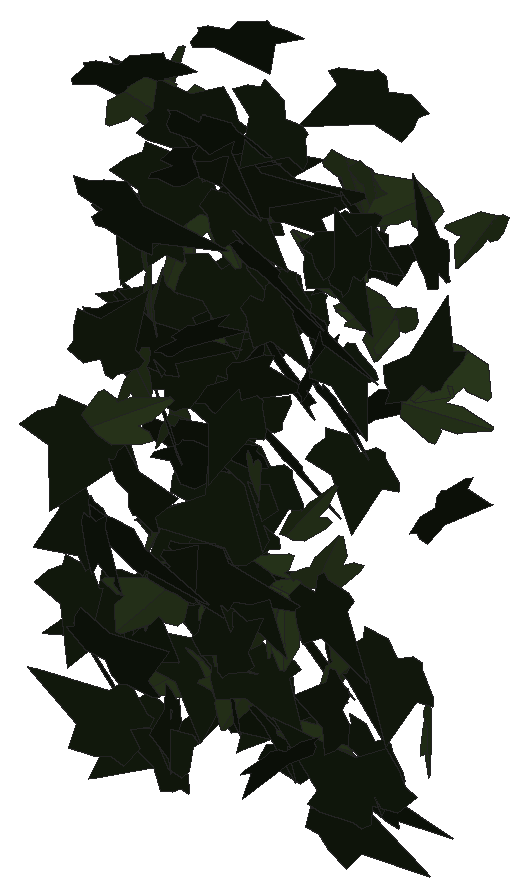
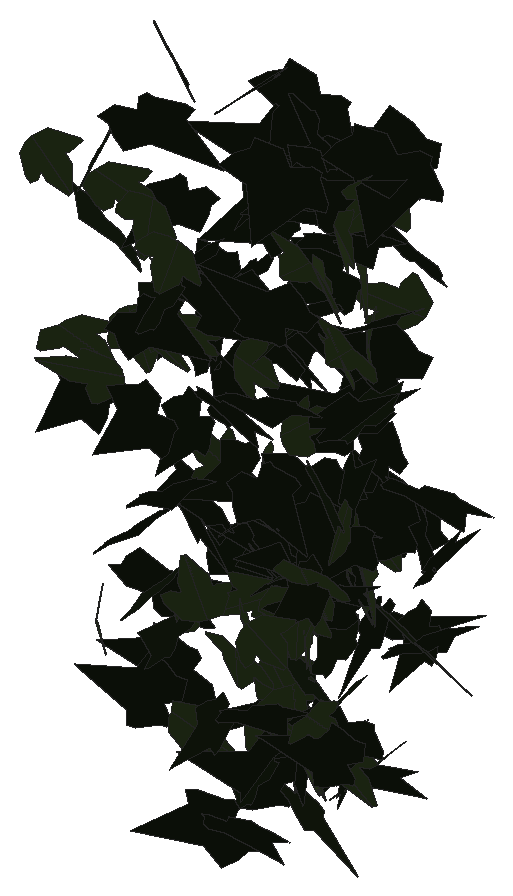
# SketchUp Ruby script. Lengths in inches.
U = 1.inch
M = Sketchup.active_model
def pt(a) = Geom::Point3d.new(a.map { |v| v * U })
def face(e, loops, mat)
  f = e.add_face(loops[0].map { |a| pt(a) })
  loops[1..].each { |l| e.add_face(l.map { |a| pt(a) }).erase! }
  f.material = f.back_material = mat if mat
  f
end
# faces: each face lists its corners as indices into pts; further lists are holes
def faces(e, pts, list, mat = nil) = list.each { |f| face(e, (f[0].is_a?(Array) ? f : [f]).map { |l| l.map { |i| pts[i] } }, mat) }
# xy, xz, yz: faces in a plane at the given z, y or x. An outline is a flat list of corners, or four numbers for a rectangle; further outlines are holes
def ring(l) = l.size == 4 ? [[l[0], l[1]], [l[2], l[1]], [l[2], l[3]], [l[0], l[3]]] : l.each_slice(2).to_a
def flat(e, list, mat, &to3) = list.each { |f| face(e, (f[0].is_a?(Array) ? f : [f]).map { |l| ring(l).map { |u, v| to3.(u, v) } }, mat) }
def xy(e, z, list, mat = nil) = flat(e, list, mat) { |x, y| [x, y, z] }
def xz(e, y, list, mat = nil) = flat(e, list, mat) { |x, z| [x, y, z] }
def yz(e, x, list, mat = nil) = flat(e, list, mat) { |y, z| [x, y, z] }
def lines(e, pts, list) = list.each { |a, b| e.add_line(pt(pts[a]), pt(pts[b])) }
# prism: a flat outline (further loops are holes) pulled along v
def prism(e, loops, v, mat = nil)
  f = face(e, loops, mat); d = Geom::Vector3d.new(v.map { |x| x * U })
  f.pushpull(f.normal.samedirection?(d) ? d.length : -d.length)
end
def box(e, o, s, mat = nil) = prism(e, [[o, [o[0] + s[0], o[1], o[2]], [o[0] + s[0], o[1] + s[1], o[2]], [o[0], o[1] + s[1], o[2]]]], [0, 0, s[2]], mat)
def at(x, y, z, deg = 0) = Geom::Transformation.translation(pt([x, y, z])) * Geom::Transformation.rotation(ORIGIN, Z_AXIS, deg.degrees)
def axes(o, x, y, z) = Geom::Transformation.new([*x, 0, *y, 0, *z, 0, *pt(o).to_a, 1])
def part(name) = M.definitions.add(name)
# library, detail: a bought-in or finely detailed component or shape, given as its bounding box
def library(name, o, s) = part(name).tap { |d| box(d.entities, o, s) }
def detail(e, o, s) = box(e.add_group.entities, o, s)
def put(e, d, t, mat = nil) = e.add_instance(d, t).tap { |i| i.material = mat if mat }
def group(e, t, mat = nil) = e.add_group.tap { |g| g.transformation = t; g.material = mat if mat }.entities
root = M.entities
M.materials.add("1026 AP 7946 SUNNY SIDE UP").color = [254, 231, 186]
M.materials.add("efeu1").color = [18, 25, 13]
M.materials.add("efeu2").color = [43, 57, 29]
c1 = part("ivyleaf_9")
p = [[1.54,2.16,1.25],[1.36,2.04,1.19],[-0.21,0.99,0.68],[-0.71,1.11,0.82],[-0.85,0.86,0.67],[-0.8,0.17,0.21],
  [-0.9,-0.01,0.1],[-0.67,-0.16,-0.02],[-0.08,-0.08,-0.05],[-0.03,-0.6,-0.4],[0.65,-0.88,-0.66],[0.83,-0.6,-0.49],
  [1.29,-0.42,-0.43],[1.8125,-0.07,-0.26],[1.21,0.44,0.15]]
faces(c1.entities,p,[[0,1,2,3,4,5,6,7,8,9,10,11,12,13,14]],"efeu1")
c2 = part("ivyleaf_10")
p = [[0,0.5,-0.03],[-0.0625,2.02,-0.43],[-0.19,2.01,-0.46],[-0.54,1.05,-0.29],[-0.52,0.625,-0.18],[-0.83,0.76,-0.28],
  [-1.16,0.64,-0.33],[-1.15,0.33,-0.24],[-0.77,-0.39,0.02],[-0.3,-0.51,0.16],[0.04,-0.48,0.23],[-0.02,2.01,-0.4375],
  [-0.06,2.01,-0.43],[0.04,-0.49,0.23],[0.67,-0.49,0.14],[1.38,0.36,-0.2],[1.375,0.51,-0.24],[0.81,0.65,-0.19],
  [0.62,0.59,-0.15],[0.6,1.09,-0.28],[0.5,1.23,-0.31]]
faces(c2.entities,p,[[0,1,2,3,4,5,6,7,8,9,10],[11,12,0,13,14,15,16,17,18,19,20]],"efeu2")
put(root,c1,axes([146.34,207.53,282.68],[-0.11458,-0.05735,0.44093],[0.46004,-0.32624,0.00437],[0.50012,0.28696,0.097]),"1026 AP 7946 SUNNY SIDE UP")
put(root,c2,axes([146.33,207.56,286.51],[-0.17998,-0.16825,0.34031],[0.22211,0.30092,0.20948],[-0.54038,0.17972,-0.02724]),"1026 AP 7946 SUNNY SIDE UP")
put(root,c1,axes([146.125,207.66,287.49],[-0.35598,0.26157,0.18173],[0.20681,-0.1171,0.35508],[0.44949,0.26103,-0.01945]),"1026 AP 7946 SUNNY SIDE UP")
put(root,c1,axes([146.3,207.96,281.36],[-0.37631,-0.28963,-0.13625],[-0.16376,-0.08298,0.38565],[-0.47198,0.25971,-0.02517]),"1026 AP 7946 SUNNY SIDE UP")
put(root,c1,axes([149.12,208.05,281.89],[-0.08149,0.34391,-0.18116],[0.03588,-0.17637,-0.35931],[-0.6077,-0.05653,0.00308]),"1026 AP 7946 SUNNY SIDE UP")
put(root,c1,axes([145.72,208.29,289.42],[0.35847,-0.07858,0.41361],[0.57645,-0.16589,-0.2486],[0.28705,0.43128,-0.01728]),"1026 AP 7946 SUNNY SIDE UP")
put(root,c2,axes([146.45,208.48,283.31],[-0.42331,-0.17634,0.21143],[-0.22299,-0.15626,-0.32925],[0.36376,-0.30099,0.04422]),"1026 AP 7946 SUNNY SIDE UP")
put(root,c1,axes([145.78,208.74,284.66],[0.02851,0.01116,0.39344],[0.25825,-0.34537,0.00034],[0.54233,0.16388,-0.02085]),"1026 AP 7946 SUNNY SIDE UP")
put(root,c1,axes([145.14,208.58,282.01],[0.47396,-0.14013,-0.18759],[-0.2741,0.05421,-0.34142],[0.23386,0.34755,-0.01997]),"1026 AP 7946 SUNNY SIDE UP")
put(root,c1,axes([144.9375,208.9,283.82],[0.04348,-0.10932,-0.40963],[0.628,-0.08975,0.0536],[-0.15764,-0.38772,0.10052]),"1026 AP 7946 SUNNY SIDE UP")
put(root,c1,axes([149.72,208.57,282.58],[-0.10359,-0.01043,-0.40068],[-0.60269,0.06915,0.06539],[0.10455,0.38831,-0.02006]),"1026 AP 7946 SUNNY SIDE UP")
put(root,c1,axes([145.39,208.82,283.78],[0.45446,-0.18086,0.27953],[0.33247,-0.17388,-0.35111],[0.39211,0.35705,-0.02627]),"1026 AP 7946 SUNNY SIDE UP")
put(root,c1,axes([150.02,208.46,289.85],[-0.01429,0.13954,0.37864],[-0.11431,0.3599,-0.14082],[-0.60633,-0.07114,0.01762]),"1026 AP 7946 SUNNY SIDE UP")
put(root,c1,axes([144.58,209.23,283.5],[-0.14243,-0.16436,0.36457],[-0.23731,-0.32131,-0.1949],[0.56724,-0.17569,0.01001]),"1026 AP 7946 SUNNY SIDE UP")
put(root,c1,axes([149.98,208.89,281.04],[0.00757,0.06868,0.46089],[-0.63803,0.19805,-0.02569],[-0.314,-0.40076,0.06331]),"1026 AP 7946 SUNNY SIDE UP")
put(root,c1,axes([146.72,208.68,287.51],[0.29215,0.21801,0.26175],[0.23418,0.20485,-0.29351],[-0.46982,0.23767,0.01647]),"1026 AP 7946 SUNNY SIDE UP")
put(root,c2,axes([145.72,208.93,286.54],[0.00431,-0.31487,-0.22093],[0.08161,0.21099,-0.3199],[0.59185,-0.0268,0.04572]),"1026 AP 7946 SUNNY SIDE UP")
put(root,c2,axes([146.13,208.85,287.75],[-0.04394,0.12117,0.3695],[-0.38677,0.2667,-0.11121],[-0.45118,-0.24042,0.05935]),"1026 AP 7946 SUNNY SIDE UP")
put(root,c1,axes([144.625,209.42,282.35],[-0.27092,-0.36562,0.1011],[-0.02765,-0.10225,-0.41607],[0.59547,-0.17109,0.02668]),"1026 AP 7946 SUNNY SIDE UP")
put(root,c1,axes([147.29,209.32,286.38],[-0.51987,-0.00879,-0.25074],[0.37992,-0.06273,-0.33623],[-0.04748,-0.4057,0.05499]),"1026 AP 7946 SUNNY SIDE UP")
put(root,c1,axes([145.4,209.21,282.45],[-0.57652,0.24626,0.03011],[-0.06689,-0.01359,-0.45366],[-0.3839,-0.36745,0.03384]),"1026 AP 7946 SUNNY SIDE UP")
put(root,c1,axes([144.55,209.45,284.92],[-0.58467,-0.19631,-0.09866],[0.17905,-0.01539,-0.42803],[0.29219,-0.38338,0.06487]),"1026 AP 7946 SUNNY SIDE UP")
put(root,c1,axes([149,209.34,280.32],[0.20714,-0.07694,-0.41271],[0.594,0.18077,0.09336],[0.24029,-0.38055,0.12497]),"1026 AP 7946 SUNNY SIDE UP")
put(root,c1,axes([145.63,209.11,282.32],[0.18332,-0.11785,-0.43679],[-0.43229,0.32209,-0.16849],[0.539,0.29841,0.01342]),"1026 AP 7946 SUNNY SIDE UP")
put(root,c2,axes([145.73,209.52,282.94],[0.31557,-0.29001,0.16499],[0.11435,-0.14609,-0.36353],[0.50952,0.21241,-0.0206]),"1026 AP 7946 SUNNY SIDE UP")
put(root,c1,axes([146.67,209.25,290.72],[0.63521,0.10103,-0.0912],[-0.12008,-0.06027,-0.42745],[-0.17449,0.40927,-0.03784]),"1026 AP 7946 SUNNY SIDE UP")
put(root,c1,axes([149.5,209.64,281.48],[0.02809,-0.33997,0.1459],[0.00465,-0.14359,-0.35153],[0.58025,0.01761,-0.00424]),"1026 AP 7946 SUNNY SIDE UP")
put(root,c1,axes([145.15,209.4,286.65],[0.18157,-0.04685,0.45099],[0.65903,-0.12779,-0.12865],[0.21335,0.43461,0.01358]),"1026 AP 7946 SUNNY SIDE UP")
put(root,c1,axes([146.45,209.58,290.3125],[-0.01147,-0.02937,-0.4212],[0.64309,0.02428,-0.00918],[0.03909,-0.40803,0.02737]),"1026 AP 7946 SUNNY SIDE UP")
put(root,c1,axes([148.47,209.62,283.52],[-0.07092,-0.10751,-0.41748],[0.65506,0.02896,-0.0556],[0.06549,-0.40611,0.10401]),"1026 AP 7946 SUNNY SIDE UP")
put(root,c1,axes([147.11,209.5625,288.78],[0.62479,-0.1759,0.05333],[0.05181,-0.05544,-0.44635],[0.28407,0.39698,-0.03588]),"1026 AP 7946 SUNNY SIDE UP")
put(root,c1,axes([146.76,209.52,282.07],[-0.22697,0.28518,0.24524],[0.20555,-0.19821,0.32736],[0.54502,0.19352,-0.02133]),"1026 AP 7946 SUNNY SIDE UP")
put(root,c1,axes([146.93,209.49,289.71],[0.24049,0.01486,0.39247],[0.59898,-0.02046,-0.15688],[0.02118,0.40993,-0.01965]),"1026 AP 7946 SUNNY SIDE UP")
put(root,c1,axes([146.96,209.52,289.54],[0.21222,-0.27332,-0.30954],[-0.16993,0.27935,-0.31178],[0.61379,0.17184,0.02071]),"1026 AP 7946 SUNNY SIDE UP")
put(root,c1,axes([146.2,209.55,283.26],[0.31222,0.08967,-0.4258],[0.53074,0.24246,0.22238],[0.40201,-0.38974,0.0371]),"1026 AP 7946 SUNNY SIDE UP")
put(root,c1,axes([147.13,209.32,286.7],[-0.04177,0.09236,-0.41009],[-0.08616,0.39503,0.10037],[0.63756,0.05943,-0.0133]),"1026 AP 7946 SUNNY SIDE UP")
put(root,c1,axes([146.06,209.4,283.25],[0.13493,0.18267,-0.38061],[0.16325,0.35672,0.20804],[0.62868,-0.13184,0.02766]),"1026 AP 7946 SUNNY SIDE UP")
put(root,c1,axes([149.62,209.97,282.71],[-0.11211,-0.40787,0.12598],[-0.02984,-0.12317,-0.42727],[0.66993,-0.07374,0.00205]),"1026 AP 7946 SUNNY SIDE UP")
put(root,c1,axes([147.5,210.05,290.75],[-0.22523,-0.2758,0.27981],[-0.10509,-0.26931,-0.31779],[0.60128,-0.15038,0.04927]),"1026 AP 7946 SUNNY SIDE UP")
put(root,c1,axes([145.6,209.93,279.74],[0.06804,-0.34981,-0.06883],[0.02076,-0.06368,0.36271],[-0.55903,-0.04494,0.00509]),"1026 AP 7946 SUNNY SIDE UP")
put(root,c1,axes([145.41,209.98,280.12],[-0.50858,-0.1978,0.12312],[-0.13387,-0.0912,-0.38973],[0.33882,-0.33294,0.03083]),"1026 AP 7946 SUNNY SIDE UP")
put(root,c1,axes([146.71,209.86,283.25],[-0.1452,-0.07776,-0.41071],[0.61179,0.09888,-0.11226],[0.18098,-0.39665,0.04998]),"1026 AP 7946 SUNNY SIDE UP")
put(root,c2,axes([145.42,209.74,283.48],[0.18911,-0.35834,-0.13358],[-0.06344,0.12109,-0.38869],[0.59476,0.12686,0.00101]),"1026 AP 7946 SUNNY SIDE UP")
put(root,c2,axes([145.02,210.0625,287.42],[0.06252,-0.10645,0.39735],[0.40863,-0.28864,-0.11118],[0.4796,0.25981,0.04294]),"1026 AP 7946 SUNNY SIDE UP")
put(root,c1,axes([147.42,209.76,287.85],[0.18573,-0.26181,-0.23419],[-0.13911,0.20783,-0.29465],[0.52557,0.14753,0.00477]),"1026 AP 7946 SUNNY SIDE UP")
put(root,c1,axes([145.58,210.13,289.125],[-0.43309,-0.29961,-0.01191],[0.03845,-0.00912,-0.41857],[0.46979,-0.27545,0.02328]),"1026 AP 7946 SUNNY SIDE UP")
put(root,c1,axes([146.95,210.1,284],[-0.51564,-0.01116,0.29046],[-0.43109,-0.09008,-0.33262],[0.1054,-0.42303,0.06057]),"1026 AP 7946 SUNNY SIDE UP")
put(root,c1,axes([145.42,210.21,279.96],[-0.0198,-0.03089,0.41541],[-0.17984,-0.38688,-0.03646],[0.61024,-0.11501,0.00274]),"1026 AP 7946 SUNNY SIDE UP")
put(root,c2,axes([147.93,209.87,284.35],[-0.00619,-0.29915,0.21667],[0.02685,0.21166,0.30921],[-0.57592,0.01309,0.01209]),"1026 AP 7946 SUNNY SIDE UP")
put(root,c2,axes([148.33,210.28,281.96],[-0.01656,0.04386,0.39384],[0.2344,-0.35184,0.04379],[0.5574,0.14926,-0.00671]),"1026 AP 7946 SUNNY SIDE UP")
put(root,c1,axes([145.85,209.71,289.59],[0.40829,0.1815,0.33611],[0.39514,0.20724,-0.32462],[-0.43223,0.3609,0.02072]),"1026 AP 7946 SUNNY SIDE UP")
put(root,c1,axes([145.73,210.3125,283.14],[-0.39581,-0.23494,0.13572],[-0.10522,-0.12198,-0.35297],[0.41132,-0.25728,0.04031]),"1026 AP 7946 SUNNY SIDE UP")
put(root,c1,axes([150.28,209.74,287.62],[-0.51887,0.3022,-0.16496],[-0.1532,0.1327,0.46069],[0.5168,0.34275,-0.02905]),"1026 AP 7946 SUNNY SIDE UP")
put(root,c1,axes([144.82,210.43,286.4],[-0.04605,-0.30692,0.30359],[0.12614,-0.2958,-0.30907],[0.65899,0.03517,0.08037]),"1026 AP 7946 SUNNY SIDE UP")
put(root,c1,axes([144.8,210.4,288.04],[-0.26732,-0.32537,0.1346],[-0.00014,-0.14716,-0.37326],[0.55241,-0.15749,0.06504]),"1026 AP 7946 SUNNY SIDE UP")
put(root,c1,axes([147.67,210.15,287.62],[0.49542,-0.16371,0.15009],[0.17755,-0.09928,-0.36475],[0.29646,0.33303,-0.03237]),"1026 AP 7946 SUNNY SIDE UP")
put(root,c1,axes([145.54,209.9,285.8],[-0.08118,-0.01082,0.47744],[0.69708,0.13539,0.05492],[-0.21343,0.44629,-0.00223]),"1026 AP 7946 SUNNY SIDE UP")
put(root,c1,axes([146.34,210.34,283.21],[-0.1239,-0.37337,0.02053],[0.00451,-0.02314,-0.39318],[0.5881,-0.07849,0.00734]),"1026 AP 7946 SUNNY SIDE UP")
put(root,c1,axes([144.66,209.92,290.6875],[0.4097,0.37246,-0.04317],[-0.00625,-0.05085,-0.46782],[-0.5897,0.25931,-0.02503]),"1026 AP 7946 SUNNY SIDE UP")
put(root,c1,axes([148.84,210.21,280.21],[0.31191,-0.14366,0.30606],[0.39216,-0.16318,-0.2531],[0.34156,0.31854,0.0111]),"1026 AP 7946 SUNNY SIDE UP")
put(root,c1,axes([146.17,210.05,284.92],[0.2308,0.34443,-0.20631],[-0.14802,-0.17954,-0.38647],[-0.61033,0.17379,0.01571]),"1026 AP 7946 SUNNY SIDE UP")
put(root,c1,axes([146.21,210.28,287.71],[-0.10006,-0.36587,-0.08568],[0.03329,0.07861,-0.38204],[0.58831,-0.06668,0.00704]),"1026 AP 7946 SUNNY SIDE UP")
put(root,c2,axes([147.125,209.89,284.6875],[0.05639,-0.00494,-0.37387],[-0.10393,0.35847,-0.00966],[0.56111,0.06689,0.03579]),"1026 AP 7946 SUNNY SIDE UP")
put(root,c1,axes([145.41,210.18,284.74],[0.04865,-0.25975,0.32765],[-0.02529,0.31941,0.27098],[-0.64699,-0.03202,0.01404]),"1026 AP 7946 SUNNY SIDE UP")
put(root,c2,axes([145.97,210.36,288.62],[0.43712,-0.00819,0.25615],[0.38455,-0.05972,-0.28401],[0.07209,0.36819,-0.03816]),"1026 AP 7946 SUNNY SIDE UP")
put(root,c2,axes([144.74,210.14,290.125],[-0.29255,-0.21772,-0.27913],[0.30097,0.19068,-0.29347],[0.4544,-0.26647,0.01467]),"1026 AP 7946 SUNNY SIDE UP")
put(root,c1,axes([147.81,210.36,286.51],[0.06363,0.2968,0.2719],[-0.22334,-0.2352,0.29543],[0.58133,-0.12285,0.08374]),"1026 AP 7946 SUNNY SIDE UP")
put(root,c2,axes([149.65,210.63,281.44],[0.13475,-0.15519,0.3516],[0.37062,-0.2511,-0.17961],[0.46007,0.24774,0.04171]),"1026 AP 7946 SUNNY SIDE UP")
put(root,c1,axes([145.64,210.48,289.71],[0.11405,0.03258,0.43799],[-0.65861,0.08523,0.06741],[-0.12404,-0.42261,0.04477]),"1026 AP 7946 SUNNY SIDE UP")
put(root,c1,axes([145.125,210.73,282.49],[0.03648,-0.22379,0.30587],[0.11636,-0.29005,-0.23189],[0.57456,0.07295,0.02754]),"1026 AP 7946 SUNNY SIDE UP")
put(root,c2,axes([146.85,210.67,282.43],[0.2914,-0.204,0.27077],[0.26313,-0.20441,-0.28495],[0.45384,0.2495,-0.00864]),"1026 AP 7946 SUNNY SIDE UP")
put(root,c2,axes([146.36,210.59,281.77],[-0.1763,-0.36558,0.11075],[-0.05154,-0.10457,-0.39454],[0.59789,-0.11681,-0.00135]),"1026 AP 7946 SUNNY SIDE UP")
put(root,c1,axes([148.08,210.63,286.86],[0.07974,-0.37103,-0.04874],[-0.02532,0.04341,-0.3854],[0.58718,0.05226,-0.01]),"1026 AP 7946 SUNNY SIDE UP")
put(root,c1,axes([145.63,210.73,283.9],[0.02391,-0.40017,0.06371],[0.08147,-0.06171,-0.40984],[0.63203,0.02309,0.05042]),"1026 AP 7946 SUNNY SIDE UP")
put(root,c1,axes([146.63,210.8125,284.42],[-0.06908,-0.39553,0.14656],[-0.02546,-0.1436,-0.41081],[0.66165,-0.04682,-0.00051]),"1026 AP 7946 SUNNY SIDE UP")
put(root,c1,axes([146.99,210.78,286.08],[0.02503,-0.12268,0.37408],[0.18453,-0.34514,-0.1272],[0.57481,0.11614,0.02455]),"1026 AP 7946 SUNNY SIDE UP")
put(root,c1,axes([145.16,210.82,286.4],[-0.19441,-0.01128,0.41962],[-0.50008,-0.26354,-0.1085],[0.40071,-0.33436,0.06818]),"1026 AP 7946 SUNNY SIDE UP")
put(root,c2,axes([145.15,210.52,287.24],[0.42626,-0.24979,0.02834],[-0.00455,0.03944,0.37897],[-0.39536,-0.26976,0.0262]),"1026 AP 7946 SUNNY SIDE UP")
put(root,c2,axes([146.37,210.69,280.91],[-0.29885,-0.30964,0.15079],[-0.05729,-0.15017,-0.37241],[0.53668,-0.18845,0.04422]),"1026 AP 7946 SUNNY SIDE UP")
put(root,c1,axes([145.46,210.77,280.95],[-0.17974,-0.37065,-0.02442],[0.03229,0.01625,-0.3992],[0.58291,-0.11519,0.01458]),"1026 AP 7946 SUNNY SIDE UP")
put(root,c1,axes([148.25,210.37,289.03],[0.02449,-0.09265,-0.38901],[-0.08704,0.373,-0.09459],[0.60432,0.05748,0.00214]),"1026 AP 7946 SUNNY SIDE UP")
put(root,c1,axes([148.04,210.83,281.86],[0.23849,-0.38022,0.15111],[0.05595,-0.14586,-0.42208],[0.63959,0.15453,-0.01942]),"1026 AP 7946 SUNNY SIDE UP")
put(root,c2,axes([146.6875,210.43,282.84],[0.11995,0.17873,0.33999],[0.28528,0.27607,-0.19622],[-0.51501,0.19456,-0.02951]),"1026 AP 7946 SUNNY SIDE UP")
put(root,c2,axes([145.74,210.94,286.15],[-0.01791,0.03835,0.40778],[0.08621,-0.39183,0.03846],[0.619,0.05568,0.00644]),"1026 AP 7946 SUNNY SIDE UP")
put(root,c1,axes([149.9,210.54,288.97],[-0.1237,-0.25634,0.33431],[0.10643,0.31939,0.27745],[-0.6433,0.10213,-0.01838]),"1026 AP 7946 SUNNY SIDE UP")
put(root,c2,axes([145.29,210.65,280.82],[0.51079,-0.03216,-0.23614],[-0.348,0.07148,-0.33329],[0.10563,0.39099,0.04389]),"1026 AP 7946 SUNNY SIDE UP")
put(root,c1,axes([150.06,210.36,285.2],[-0.07317,0.09051,-0.39385],[-0.2249,0.35521,0.1065],[0.57621,0.15013,-0.00845]),"1026 AP 7946 SUNNY SIDE UP")
put(root,c1,axes([146.32,210.71,281.25],[0.05039,-0.33339,-0.21647],[0.1435,0.20952,-0.32989],[0.60118,-0.02207,0.09688]),"1026 AP 7946 SUNNY SIDE UP")
put(root,c1,axes([146.8,210.71,284.98],[0.51576,-0.19119,0.02795],[0.01145,-0.04332,-0.38984],[0.30367,0.32636,-0.03277]),"1026 AP 7946 SUNNY SIDE UP")
put(root,c2,axes([147.95,210.76,280.39],[-0.12506,0.05293,0.38657],[-0.59406,-0.03686,-0.07742],[0.04004,-0.38151,0.05882]),"1026 AP 7946 SUNNY SIDE UP")
put(root,c1,axes([145.11,210.64,284.62],[0.57652,0.16465,-0.07071],[-0.07421,-0.06396,-0.41254],[-0.27109,0.36767,-0.03745]),"1026 AP 7946 SUNNY SIDE UP")
put(root,c1,axes([145.45,210.79,283.24],[-0.12963,-0.27226,-0.27299],[0.14208,0.2477,-0.29139],[0.57851,-0.12184,0.0104]),"1026 AP 7946 SUNNY SIDE UP")
put(root,c1,axes([145.88,210.68,280.78],[0.29004,-0.08001,-0.33272],[-0.49928,0.06627,-0.20364],[0.15399,0.36558,-0.03359]),"1026 AP 7946 SUNNY SIDE UP")
put(root,c2,axes([144.72,210.9,287.85],[0.46324,-0.02942,0.26968],[0.39594,-0.08472,-0.30206],[0.12253,0.385,-0.04348]),"1026 AP 7946 SUNNY SIDE UP")
put(root,c1,axes([147.73,210.87,288.35],[0.1339,-0.35831,-0.17316],[-0.07295,0.15961,-0.37839],[0.61666,0.09669,-0.00717]),"1026 AP 7946 SUNNY SIDE UP")
put(root,c1,axes([144.85,210.94,281.94],[0.22389,-0.35222,-0.05992],[-0.06153,0.04468,-0.39062],[0.55745,0.1464,-0.01905]),"1026 AP 7946 SUNNY SIDE UP")
put(root,c2,axes([144.98,210.65,284.84],[-0.00818,-0.22421,-0.31245],[0.04665,0.30086,-0.22886],[0.58961,-0.02691,0.01377]),"1026 AP 7946 SUNNY SIDE UP")
put(root,c2,axes([146.73,211,282.05],[0.54505,-0.07496,0.13016],[0.17704,-0.07407,-0.36273],[0.14926,0.36158,-0.04503]),"1026 AP 7946 SUNNY SIDE UP")
put(root,c1,axes([145.73,210.96,282.28],[-0.42084,0.25878,-0.04771],[0.02535,-0.0519,-0.3829],[-0.413,-0.26687,0.02511]),"1026 AP 7946 SUNNY SIDE UP")
put(root,c1,axes([146.22,211.22,280.17],[0.18499,-0.30386,0.18308],[0.07015,-0.17482,-0.33614],[0.55043,0.12441,-0.01869]),"1026 AP 7946 SUNNY SIDE UP")
put(root,c1,axes([145.59,211,280.06],[-0.3809,0.29247,-0.04882],[0.02458,-0.05066,-0.39098],[-0.46565,-0.24191,0.0193]),"1026 AP 7946 SUNNY SIDE UP")
put(root,c2,axes([145.65,211.03,283.3],[-0.60615,0.1046,0.0467],[-0.08735,-0.03513,-0.4087],[-0.1561,-0.38649,0.04734]),"1026 AP 7946 SUNNY SIDE UP")
put(root,c2,axes([145.66,211.1,281.86],[0.23247,0.35661,-0.077],[-0.07949,-0.062,-0.39738],[-0.56804,0.15462,0.0241]),"1026 AP 7946 SUNNY SIDE UP")
put(root,c2,axes([147.34,211.14,282.75],[-0.22299,-0.34414,0.03781],[0.01054,0.03904,0.38358],[-0.54442,0.14171,-0.00806]),"1026 AP 7946 SUNNY SIDE UP")
put(root,c2,axes([148.95,211.29,289.41],[-0.29954,-0.11083,0.29462],[-0.2699,-0.24133,-0.21508],[0.40079,-0.24535,0.07535]),"1026 AP 7946 SUNNY SIDE UP")
put(root,c2,axes([150.23,211.27,289.48],[-0.14037,-0.33356,0.15916],[-0.05833,-0.15195,-0.3566],[0.57633,-0.09662,0.00267]),"1026 AP 7946 SUNNY SIDE UP")
put(root,c1,axes([146.02,210.94,280.17],[0.17077,0.0337,0.39606],[0.58964,0.08432,-0.11631],[-0.14213,0.39031,-0.00667]),"1026 AP 7946 SUNNY SIDE UP")
put(root,c1,axes([147.47,211.07,285.84],[0.51403,-0.11328,-0.14825],[-0.22637,0.02092,-0.35535],[0.17671,0.35631,-0.02397]),"1026 AP 7946 SUNNY SIDE UP")
put(root,c2,axes([145.22,211.28,284.04],[0.56961,-0.04363,-0.04417],[-0.07226,-0.02643,-0.37464],[0.06307,0.36379,-0.03035]),"1026 AP 7946 SUNNY SIDE UP")
put(root,c2,axes([144.5,211.39,290.1],[0.18223,-0.30514,0.18536],[0.15124,-0.15697,-0.33577],[0.53752,0.14762,0.03164]),"1026 AP 7946 SUNNY SIDE UP")
put(root,c1,axes([144.62,211.13,281.69],[0.44892,0.17121,-0.11202],[-0.12268,-0.08239,-0.34213],[-0.29526,0.29455,-0.02815]),"1026 AP 7946 SUNNY SIDE UP")
put(root,c1,axes([148.25,211.41,290.85],[0.06133,0.04028,-0.39813],[-0.28266,-0.34272,-0.05746],[-0.54204,0.18328,-0.01508]),"1026 AP 7946 SUNNY SIDE UP")
put(root,c2,axes([145.4,211.05,282.89],[0.04653,-0.03769,-0.3647],[-0.13287,0.34411,-0.04303],[0.54345,0.08736,0.02071]),"1026 AP 7946 SUNNY SIDE UP")
put(root,c2,axes([148.41,211.38,287.28],[-0.25165,-0.33855,0.07086],[-0.02351,-0.07106,-0.38582],[0.54331,-0.15988,0.01612]),"1026 AP 7946 SUNNY SIDE UP")
put(root,c2,axes([149.05,211.25,286.1],[-0.05138,-0.04222,-0.37075],[0.56765,0.02437,-0.03659],[0.04441,-0.3603,0.03882]),"1026 AP 7946 SUNNY SIDE UP")
put(root,c1,axes([147.71,211.52,284.72],[-0.17877,-0.35834,0.01567],[0.01041,-0.02019,-0.3872],[0.56401,-0.11321,0.01211]),"1026 AP 7946 SUNNY SIDE UP")
put(root,c1,axes([145.04,211.34,283.96],[0.50889,-0.15824,-0.08656],[-0.1407,0.00543,-0.36949],[0.24331,0.3341,-0.03261]),"1026 AP 7946 SUNNY SIDE UP")
put(root,c2,axes([149.47,211.57,286.83],[0.39544,0.15955,-0.24225],[-0.28149,-0.15647,-0.30634],[-0.34854,0.30739,-0.02745]),"1026 AP 7946 SUNNY SIDE UP")
put(root,c2,axes([148.25,211.36,287.24],[0.20931,-0.10846,-0.32829],[-0.42909,0.16474,-0.17457],[0.30834,0.30288,-0.02008]),"1026 AP 7946 SUNNY SIDE UP")
put(root,c1,axes([146.14,211.22,284.78],[-0.48972,0.12981,-0.17105],[-0.21898,0.09735,0.34655],[0.24995,0.33961,-0.03152]),"1026 AP 7946 SUNNY SIDE UP")
put(root,c1,axes([145.87,211.65,286.94],[-0.40836,-0.28158,-0.09727],[0.18377,0.01618,-0.38733],[0.42844,-0.27532,0.07342]),"1026 AP 7946 SUNNY SIDE UP")
put(root,c2,axes([144.74,211.56,289.38],[0.33385,-0.29989,0.05143],[0.02087,-0.05376,-0.37828],[0.47802,0.21179,-0.0194]),"1026 AP 7946 SUNNY SIDE UP")
put(root,c2,axes([147.4375,211.48,287.53],[0.31524,0.08652,0.29309],[-0.45375,-0.02377,0.21718],[0.10974,-0.34683,0.05606]),"1026 AP 7946 SUNNY SIDE UP")
put(root,c2,axes([148.06,211.48,289.3],[-0.53855,0.1419,0.03151],[-0.06318,-0.01948,-0.3805],[-0.21905,-0.34324,0.03227]),"1026 AP 7946 SUNNY SIDE UP")
put(root,c1,axes([145.55,211.7,287.98],[0.11567,-0.38428,0.03652],[-0.00023,-0.03833,-0.40322],[0.60713,0.0732,-0.00711]),"1026 AP 7946 SUNNY SIDE UP")
put(root,c1,axes([148.1,211.28,285.75],[0.25899,0.25029,0.24092],[0.24296,0.17555,-0.3065],[-0.47899,0.22437,-0.0252]),"1026 AP 7946 SUNNY SIDE UP")
put(root,c2,axes([144.84,211.77,281.27],[0.23871,-0.28508,0.1072],[0.04497,-0.1042,-0.33253],[0.47595,0.15283,-0.02235]),"1026 AP 7946 SUNNY SIDE UP")
put(root,c1,axes([145.46,211.45,290.86],[0.43296,0.30341,-0.01938],[0.00838,-0.03251,-0.42146],[-0.47811,0.27419,-0.02493]),"1026 AP 7946 SUNNY SIDE UP")
put(root,c1,axes([146.41,211.81,286.76],[-0.51429,-0.05158,-0.14833],[0.23273,-0.02381,-0.3384],[0.05887,-0.35645,0.04193]),"1026 AP 7946 SUNNY SIDE UP")
put(root,c1,axes([146.07,211.64,288.24],[0.05739,-0.01528,0.42032],[0.62025,-0.10471,-0.041],[0.16617,0.39611,0.00786]),"1026 AP 7946 SUNNY SIDE UP")
put(root,c1,axes([146.51,211.52,279.57],[0.083,0.07958,-0.37777],[0.27144,0.32416,0.09984],[0.52466,-0.1803,0.00811]),"1026 AP 7946 SUNNY SIDE UP")
put(root,c1,axes([146.55,211.67,281.34],[0.46107,-0.1718,-0.13851],[-0.16964,0.07969,-0.34938],[0.29706,0.31217,0.01546]),"1026 AP 7946 SUNNY SIDE UP")
put(root,c1,axes([145.7,211.8,285.69],[-0.10121,0.29346,-0.24875],[0.06746,-0.23942,-0.31082],[-0.59542,-0.07701,0.00707]),"1026 AP 7946 SUNNY SIDE UP")
put(root,c2,axes([145.79,212.01,287.77],[0.03965,-0.25759,0.27215],[0.03685,-0.26461,-0.26818],[0.58066,0.03438,-0.00156]),"1026 AP 7946 SUNNY SIDE UP")
put(root,c1,axes([144.72,211.52,285.73],[-0.04901,0.19671,0.29714],[-0.06713,0.28412,-0.20351],[-0.54337,-0.05284,-0.00166]),"1026 AP 7946 SUNNY SIDE UP")
put(root,c1,axes([145.74,211.99,281.9],[-0.38381,-0.2688,0.02257],[0.00167,-0.03255,-0.37351],[0.42426,-0.24304,0.02188]),"1026 AP 7946 SUNNY SIDE UP")
put(root,c1,axes([145.32,211.76,288.45],[0.01476,-0.02287,0.38213],[0.55837,-0.10931,-0.01683],[0.17301,0.35471,0.02173]),"1026 AP 7946 SUNNY SIDE UP")
put(root,c2,axes([145.59,212.02,283.27],[-0.18737,-0.2765,0.22519],[0.00353,-0.23292,-0.30148],[0.55575,-0.09175,0.07784]),"1026 AP 7946 SUNNY SIDE UP")
put(root,c1,axes([147.77,212.03,287.875],[-0.06096,0.09888,-0.36756],[-0.00223,-0.35933,-0.10438],[-0.58301,-0.00896,0.03883]),"1026 AP 7946 SUNNY SIDE UP")
put(root,c1,axes([147.24,212.16,288.24],[0.13637,-0.29807,0.24395],[0.07691,-0.23388,-0.32082],[0.5953,0.0985,-0.01444]),"1026 AP 7946 SUNNY SIDE UP")
put(root,c2,axes([144.52,212.06,282.25],[0.1747,0.21497,-0.23967],[-0.15527,-0.21211,-0.25043],[-0.47475,0.14848,-0.00629]),"1026 AP 7946 SUNNY SIDE UP")
put(root,c2,axes([147.28,211.9,289.0625],[-0.53618,0.09439,-0.04375],[0.0498,-0.04597,-0.36292],[-0.15531,-0.34061,0.03467]),"1026 AP 7946 SUNNY SIDE UP")
put(root,c1,axes([146.02,212.08,279.96],[-0.52583,-0.12112,-0.02267],[0.04482,-0.01628,-0.3656],[0.18811,-0.33469,0.02376]),"1026 AP 7946 SUNNY SIDE UP")
put(root,c1,axes([144.07,211.89,281.58],[0.28333,-0.04105,0.28382],[0.41579,-0.0788,-0.19056],[0.13881,0.31983,-0.00851]),"1026 AP 7946 SUNNY SIDE UP")
